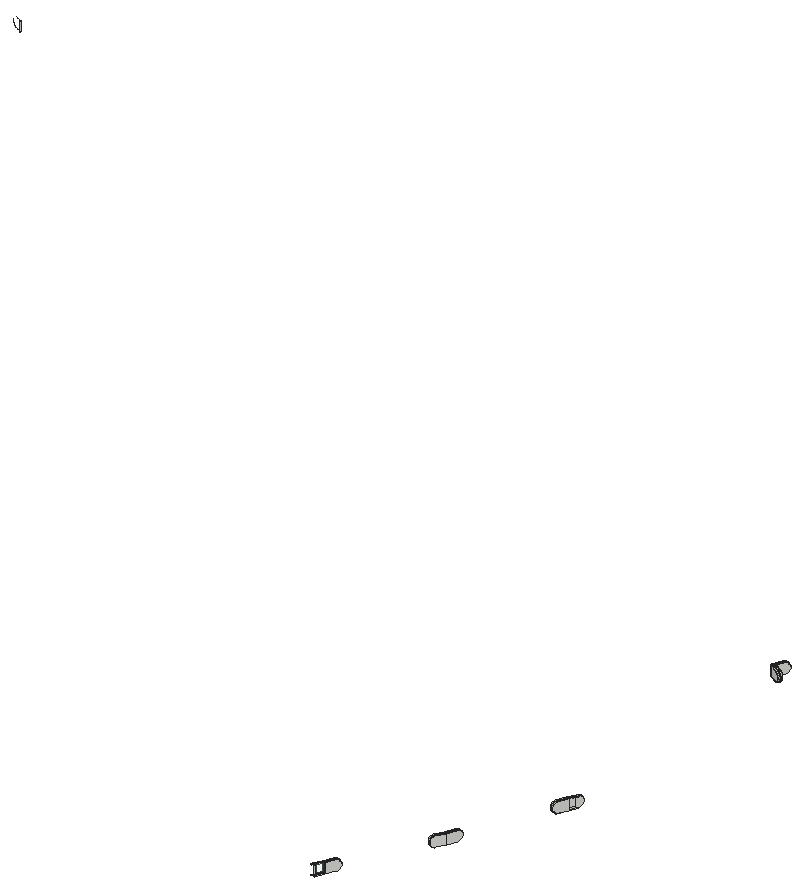
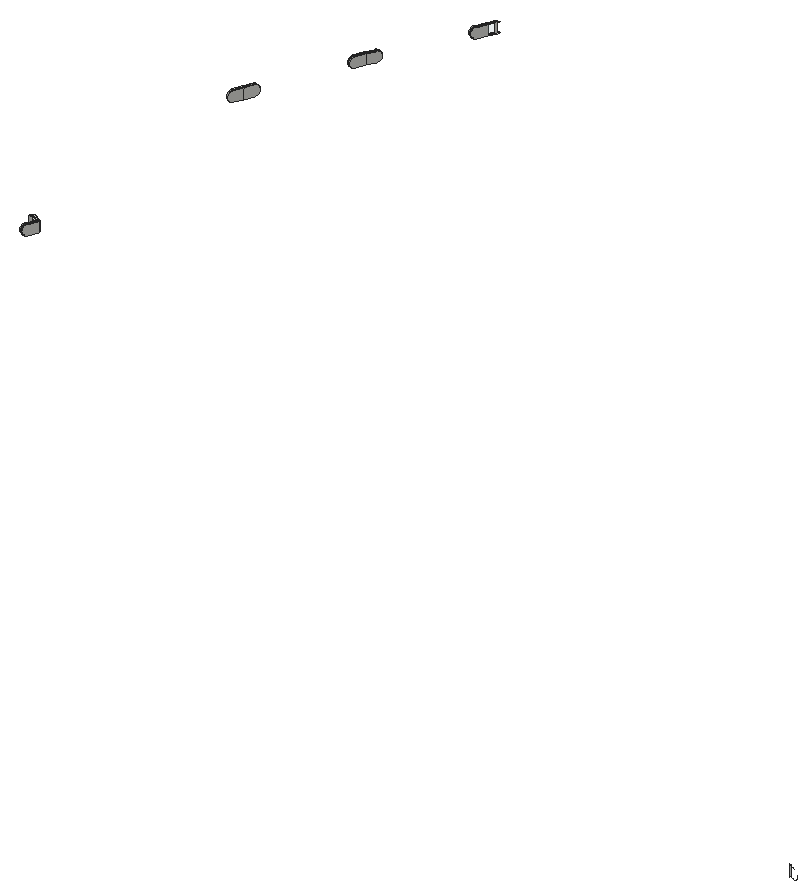
# SketchUp Ruby script. Lengths in inches.
U = 1.inch
M = Sketchup.active_model
def pt(a) = Geom::Point3d.new(a.map { |v| v * U })
def face(e, loops, mat)
  f = e.add_face(loops[0].map { |a| pt(a) })
  loops[1..].each { |l| e.add_face(l.map { |a| pt(a) }).erase! }
  f.material = f.back_material = mat if mat
  f
end
# faces: each face lists its corners as indices into pts; further lists are holes
def faces(e, pts, list, mat = nil) = list.each { |f| face(e, (f[0].is_a?(Array) ? f : [f]).map { |l| l.map { |i| pts[i] } }, mat) }
# xy, xz, yz: faces in a plane at the given z, y or x. An outline is a flat list of corners, or four numbers for a rectangle; further outlines are holes
def ring(l) = l.size == 4 ? [[l[0], l[1]], [l[2], l[1]], [l[2], l[3]], [l[0], l[3]]] : l.each_slice(2).to_a
def flat(e, list, mat, &to3) = list.each { |f| face(e, (f[0].is_a?(Array) ? f : [f]).map { |l| ring(l).map { |u, v| to3.(u, v) } }, mat) }
def xy(e, z, list, mat = nil) = flat(e, list, mat) { |x, y| [x, y, z] }
def xz(e, y, list, mat = nil) = flat(e, list, mat) { |x, z| [x, y, z] }
def yz(e, x, list, mat = nil) = flat(e, list, mat) { |y, z| [x, y, z] }
def lines(e, pts, list) = list.each { |a, b| e.add_line(pt(pts[a]), pt(pts[b])) }
# prism: a flat outline (further loops are holes) pulled along v
def prism(e, loops, v, mat = nil)
  f = face(e, loops, mat); d = Geom::Vector3d.new(v.map { |x| x * U })
  f.pushpull(f.normal.samedirection?(d) ? d.length : -d.length)
end
def box(e, o, s, mat = nil) = prism(e, [[o, [o[0] + s[0], o[1], o[2]], [o[0] + s[0], o[1] + s[1], o[2]], [o[0], o[1] + s[1], o[2]]]], [0, 0, s[2]], mat)
def at(x, y, z, deg = 0) = Geom::Transformation.translation(pt([x, y, z])) * Geom::Transformation.rotation(ORIGIN, Z_AXIS, deg.degrees)
def axes(o, x, y, z) = Geom::Transformation.new([*x, 0, *y, 0, *z, 0, *pt(o).to_a, 1])
def part(name) = M.definitions.add(name)
# library, detail: a bought-in or finely detailed component or shape, given as its bounding box
def library(name, o, s) = part(name).tap { |d| box(d.entities, o, s) }
def detail(e, o, s) = box(e.add_group.entities, o, s)
def put(e, d, t, mat = nil) = e.add_instance(d, t).tap { |i| i.material = mat if mat }
def group(e, t, mat = nil) = e.add_group.tap { |g| g.transformation = t; g.material = mat if mat }.entities
root = M.entities
M.materials.add("Glass_Safety_01").color = [204, 235, 244]
M.materials["Glass_Safety_01"].alpha = 0.1
M.materials.add("[Color_000]").color = [255, 255, 255]
xy(root,333,[[944.885,768.202,944.633,768.313,944.699,768.465,945.424,770.112,945.673,769.993],[944.452,768.392,944.2,768.503,944.993,770.305,945.245,770.194,944.519,768.544],[945.673,769.993,945.424,770.112,945.425,770.115,945.677,770.004,945.675,769.999],[945.677,770.004,945.425,770.115,946.271,771.889,946.52,771.77],[945.246,770.197,944.997,770.315,945.844,772.092,946.093,771.974],
  [954.439,788.385,954.19,788.504,954.265,788.661,955.037,790.281,955.286,790.162],[954.013,788.589,953.764,788.707,954.6,790.46,954.857,790.359,954.087,788.745],[955.297,790.187,955.04,790.287,955.76,792.12,956.016,792.019],[954.857,790.359,954.6,790.46,954.605,790.472,954.611,790.484,954.86,790.366],[954.86,790.366,954.611,790.484,955.32,792.292,955.577,792.192],
  [963.05,809.92,962.794,810.021,962.855,810.177,963.512,811.85,963.765,811.74],[962.61,810.093,962.354,810.194,963.074,812.026,963.33,811.925,962.671,810.249],[963.765,811.74,963.512,811.85,963.513,811.853,963.77,811.753,963.767,811.746],[963.77,811.753,963.513,811.853,964.298,813.655,964.551,813.545],[963.332,811.929,963.079,812.039,963.865,813.843,964.118,813.733],
  [963.328,866.978,961.618,867.953,961.755,868.193,963.309,867.306,963.464,867.217],[963.562,867.388,963.406,867.477,962.17,868.183,962.28,868.437,963.698,867.627],[962.146,868.129,961.894,868.239,961.929,868.32,962.04,868.574,962.68,870.044,962.932,869.934,962.28,868.437,962.04,868.574,961.989,868.603,961.852,868.364,961.929,868.32,962.17,868.183],[962.17,868.183,961.929,868.32,962.04,868.574,962.28,868.437],[961.713,868.317,961.46,868.428,962.246,870.232,962.499,870.122],
  [961.929,868.32,961.852,868.364,961.989,868.603,962.04,868.574]])
xy(root,333.078,[[944.791,768.673,944.611,768.752,945.245,770.194,945.335,770.154,945.424,770.112],[945.424,770.112,945.335,770.154,945.425,770.115,945.424,770.113],[945.425,770.115,945.335,770.154,945.246,770.197,945.924,771.618,946.101,771.534],[954.36,788.859,954.182,788.944,954.857,790.359,954.948,790.323,955.037,790.281],[955.04,790.287,954.948,790.323,954.86,790.366,955.433,791.825,955.616,791.753],
  [954.948,790.323,954.857,790.359,954.858,790.363,954.86,790.366],[962.9375,810.388,962.754,810.46,963.33,811.925,963.422,811.889,963.512,811.85],[963.512,811.85,963.422,811.889,963.513,811.853,963.513,811.852],[963.513,811.853,963.422,811.889,963.332,811.929,963.96,813.372,964.141,813.294],[963.122,867.412,961.755,868.193,961.803,868.278,961.894,868.239,961.929,868.32,963.22,867.583],
  [961.894,868.239,961.803,868.278,961.852,868.364,961.929,868.32],[961.803,868.278,961.713,868.317,962.342,869.761,962.522,869.683,961.929,868.32,961.852,868.364]],"Glass_Safety_01")
xy(root,335.047,[[944.791,768.673,945.424,770.112,945.335,770.154,945.245,770.194,944.611,768.752],[945.424,770.112,945.424,770.113,945.425,770.115,945.335,770.154],[945.425,770.115,946.101,771.534,945.924,771.618,945.246,770.197,945.335,770.154],[954.36,788.859,955.037,790.281,954.948,790.323,954.857,790.359,954.182,788.944],[955.04,790.287,955.616,791.753,955.433,791.825,954.86,790.366,954.948,790.323],
  [954.948,790.323,954.86,790.366,954.858,790.363,954.857,790.359],[962.9375,810.388,963.512,811.85,963.422,811.889,963.33,811.925,962.754,810.46],[963.512,811.85,963.513,811.852,963.513,811.853,963.422,811.889],[963.513,811.853,964.141,813.294,963.96,813.372,963.332,811.929,963.422,811.889],[963.122,867.412,963.22,867.583,961.929,868.32,961.894,868.239,961.803,868.278,961.755,868.193],
  [961.894,868.239,961.929,868.32,961.852,868.364,961.803,868.278],[961.803,868.278,961.852,868.364,961.929,868.32,962.522,869.683,962.342,869.761,961.713,868.317]],"Glass_Safety_01")
xy(root,335.126,[[944.885,768.202,945.673,769.993,945.424,770.112,944.699,768.465,944.633,768.313],[944.452,768.392,944.519,768.544,945.245,770.194,944.993,770.305,944.2,768.503],[945.673,769.993,945.675,769.999,945.677,770.004,945.425,770.115,945.424,770.112],[945.677,770.004,946.52,771.77,946.271,771.889,945.425,770.115],[945.246,770.197,946.093,771.974,945.844,772.092,944.997,770.315],
  [954.439,788.385,955.286,790.162,955.037,790.281,954.265,788.661,954.19,788.504],[954.013,788.589,954.087,788.745,954.857,790.359,954.6,790.46,953.764,788.707],[955.297,790.187,956.016,792.019,955.76,792.12,955.04,790.287],[954.857,790.359,954.86,790.366,954.611,790.484,954.605,790.472,954.6,790.46],[954.86,790.366,955.577,792.192,955.32,792.292,954.611,790.484],
  [963.05,809.92,963.765,811.74,963.512,811.85,962.855,810.177,962.794,810.021],[962.61,810.093,962.671,810.249,963.33,811.925,963.074,812.026,962.354,810.194],[963.765,811.74,963.767,811.746,963.77,811.753,963.513,811.853,963.512,811.85],[963.77,811.753,964.551,813.545,964.298,813.655,963.513,811.853],[963.332,811.929,964.118,813.733,963.865,813.843,963.079,812.039],
  [963.328,866.978,963.464,867.217,963.309,867.306,961.755,868.193,961.618,867.953],[963.562,867.388,963.698,867.627,962.28,868.437,962.17,868.183,963.406,867.477],[962.146,868.129,962.17,868.183,961.929,868.32,961.852,868.364,961.989,868.603,962.04,868.574,962.28,868.437,962.932,869.934,962.68,870.044,962.04,868.574,961.929,868.32,961.894,868.239],[962.17,868.183,962.28,868.437,962.04,868.574,961.929,868.32],[961.713,868.317,962.499,870.122,962.246,870.232,961.46,868.428],
  [961.929,868.32,962.04,868.574,961.989,868.603,961.852,868.364]])
p = [[944.452,768.392,333],[944.342,768.14,333.036],[944.089,768.251,333.036],[944.2,768.503,333],[945.245,770.194,335.126],[944.519,768.544,335.126],
  [944.519,768.544,333],[945.245,770.194,333],[945.245,770.194,333.078],[944.611,768.752,333.078],[944.611,768.752,335.047],[945.245,770.194,335.047],
  [945.424,770.112,333.078],[945.424,770.112,333],[945.673,769.993,333],[945.673,769.993,335.126],[945.424,770.112,335.126],[945.424,770.112,335.047],
  [945.425,770.115,333],[945.425,770.115,333.078],[945.425,770.115,335.047],[945.425,770.115,335.126],[945.677,770.004,335.126],[945.677,770.004,333],
  [945.675,769.999,335.126],[945.675,769.999,333],[946.52,771.77,333],[946.638,772.019,333.036],[946.748,772.25,333.142],[946.843,772.449,333.311],
  [946.916,772.601,333.531],[946.961,772.697,333.787],[946.977,772.73,334.0625],[946.961,772.697,334.338],[946.916,772.601,334.594],[946.843,772.449,334.814],
  [946.748,772.25,334.983],[946.638,772.019,335.089],[946.52,771.77,335.126],[946.271,771.889,335.126],[946.389,772.137,335.089],[946.5,772.369,334.983],
  [946.594,772.568,334.814],[946.667,772.72,334.594],[946.713,772.816,334.338],[946.728,772.849,334.0625],[946.713,772.816,333.787],[946.667,772.72,333.531],
  [946.594,772.568,333.311],[946.5,772.369,333.142],[946.389,772.137,333.036],[946.271,771.889,333],[944.993,770.305,333],[944.993,770.305,335.126],
  [945.246,770.197,333],[945.246,770.197,333.078],[945.246,770.197,335.047],[945.246,770.197,335.126],[944.997,770.315,335.126],[944.997,770.315,333],
  [946.093,771.974,333],[946.093,771.974,335.126],[945.924,771.618,335.047],[945.924,771.618,333.078],[945.844,772.092,335.126],[945.963,772.341,335.089],
  [946.073,772.572,334.983],[946.168,772.771,334.814],[946.24,772.923,334.594],[946.286,773.019,334.338],[946.302,773.052,334.0625],[946.286,773.019,333.787],
  [946.24,772.923,333.531],[946.168,772.771,333.311],[946.073,772.572,333.142],[945.963,772.341,333.036],[945.844,772.092,333],[946.211,772.222,333.036],
  [946.211,772.222,335.089],[946.322,772.454,334.983],[946.417,772.652,334.814],[946.489,772.805,334.594],[946.535,772.901,334.338],[946.55,772.933,334.0625],
  [946.535,772.901,333.787],[946.489,772.805,333.531],[946.417,772.652,333.311],[946.322,772.454,333.142],[955.286,790.162,335.126],[954.439,788.385,335.126],
  [954.321,788.137,335.089],[954.21,787.906,334.983],[954.116,787.707,334.814],[954.043,787.554,334.594],[953.997,787.459,334.338],[953.982,787.426,334.0625],
  [953.997,787.459,333.787],[954.043,787.554,333.531],[954.116,787.707,333.311],[954.21,787.906,333.142],[954.321,788.137,333.036],[954.439,788.385,333],
  [955.286,790.162,333],[954.19,788.504,335.126],[954.265,788.661,335.126],[954.265,788.661,333],[954.19,788.504,333],[954.072,788.256,333.036],
  [953.962,788.024,333.142],[953.867,787.826,333.311],[953.794,787.673,333.531],[953.748,787.577,333.787],[953.733,787.544,334.0625],[953.748,787.577,334.338],
  [953.794,787.673,334.594],[953.867,787.826,334.814],[953.962,788.024,334.983],[954.072,788.256,335.089],[954.013,788.589,333],[954.087,788.745,333],
  [954.857,790.359,333],[954.857,790.359,333.078],[954.857,790.359,335.047],[954.857,790.359,335.126],[954.087,788.745,335.126],[954.013,788.589,335.126],
  [953.894,788.34,335.089],[953.784,788.109,334.983],[953.689,787.91,334.814],[953.616,787.758,334.594],[953.571,787.662,334.338],[953.555,787.629,334.0625],
  [953.571,787.662,333.787],[953.616,787.758,333.531],[953.689,787.91,333.311],[953.784,788.109,333.142],[953.894,788.34,333.036],[953.764,788.707,335.126],
  [954.6,790.46,335.126],[954.6,790.46,333],[953.764,788.707,333],[953.645,788.459,333.036],[953.535,788.228,333.142],[953.44,788.029,333.311],
  [953.368,787.876,333.531],[953.322,787.78,333.787],[953.306,787.748,334.0625],[953.322,787.78,334.338],[953.368,787.876,334.594],[953.44,788.029,334.814],
  [953.535,788.228,334.983],[953.645,788.459,335.089],[955.037,790.281,333],[955.037,790.281,335.126],[955.037,790.281,335.047],[954.36,788.859,335.047],
  [954.36,788.859,333.078],[955.037,790.281,333.078],[955.04,790.287,333.078],[955.04,790.287,333],[955.297,790.187,333],[955.297,790.187,335.126],
  [955.04,790.287,335.126],[955.04,790.287,335.047],[956.016,792.019,335.126],[956.016,792.019,333],[956.117,792.275,333.036],[956.211,792.513,333.142],
  [956.291,792.718,333.311],[956.353,792.876,333.531],[956.392,792.974,333.787],[956.405,793.008,334.0625],[956.392,792.974,334.338],[956.353,792.876,334.594],
  [956.291,792.718,334.814],[956.211,792.513,334.983],[956.117,792.275,335.089],[955.76,792.12,335.126],[955.76,792.12,333],[955.616,791.753,333.078],
  [955.616,791.753,335.047],[954.86,790.366,333.078],[954.86,790.366,333],[954.611,790.484,333],[954.611,790.484,335.126],[954.86,790.366,335.126],
  [954.86,790.366,335.047],[955.577,792.192,333],[955.677,792.448,333.036],[955.771,792.686,333.142],[955.852,792.891,333.311],[955.913,793.048,333.531],
  [955.952,793.147,333.787],[955.965,793.181,334.0625],[955.952,793.147,334.338],[955.913,793.048,334.594],[955.852,792.891,334.814],[955.771,792.686,334.983],
  [955.677,792.448,335.089],[955.577,792.192,335.126],[954.605,790.472,333],[954.605,790.472,335.126],[955.32,792.292,335.126],[955.421,792.548,335.089],
  [955.515,792.787,334.983],[955.595,792.992,334.814],[955.657,793.149,334.594],[955.696,793.248,334.338],[955.709,793.282,334.0625],[955.696,793.248,333.787],
  [955.657,793.149,333.531],[955.595,792.992,333.311],[955.515,792.787,333.142],[955.421,792.548,333.036],[955.32,792.292,333],[955.86,792.376,333.036],
  [955.954,792.614,333.142],[956.035,792.819,333.311],[956.097,792.976,333.531],[956.135,793.075,333.787],[956.149,793.109,334.0625],[956.135,793.075,334.338],
  [956.097,792.976,334.594],[956.035,792.819,334.814],[955.954,792.614,334.983],[955.86,792.376,335.089],[963.05,809.92,333],[963.765,811.74,333],
  [963.765,811.74,335.126],[963.05,809.92,335.126],[962.949,809.664,335.089],[962.856,809.426,334.983],[962.775,809.221,334.814],[962.713,809.064,334.594],
  [962.675,808.965,334.338],[962.661,808.931,334.0625],[962.675,808.965,333.787],[962.713,809.064,333.531],[962.775,809.221,333.311],[962.856,809.426,333.142],
  [962.949,809.664,333.036],[962.855,810.177,335.126],[963.512,811.85,335.126],[963.512,811.85,335.047],[963.512,811.85,333.078],[963.512,811.85,333],
  [962.855,810.177,333],[962.794,810.021,333],[962.693,809.765,333.036],[962.599,809.527,333.142],[962.519,809.322,333.311],[962.457,809.164,333.531],
  [962.418,809.066,333.787],[962.405,809.032,334.0625],[962.418,809.066,334.338],[962.457,809.164,334.594],[962.519,809.322,334.814],[962.599,809.527,334.983],
  [962.693,809.765,335.089],[962.794,810.021,335.126],[962.61,810.093,333],[962.671,810.249,333],[962.671,810.249,335.126],[962.61,810.093,335.126],
  [962.51,809.837,335.089],[962.416,809.599,334.983],[962.335,809.394,334.814],[962.274,809.236,334.594],[962.235,809.138,334.338],[962.222,809.104,334.0625],
  [962.235,809.138,333.787],[962.274,809.236,333.531],[962.335,809.394,333.311],[962.416,809.599,333.142],[962.51,809.837,333.036],[962.354,810.194,335.126],
  [963.074,812.026,335.126],[963.074,812.026,333],[962.354,810.194,333],[962.253,809.938,333.036],[962.159,809.699,333.142],[962.079,809.494,333.311],
  [962.017,809.337,333.531],[961.978,809.238,333.787],[961.965,809.205,334.0625],[961.978,809.238,334.338],[962.017,809.337,334.594],[962.079,809.494,334.814],
  [962.159,809.699,334.983],[962.253,809.938,335.089],[963.33,811.925,335.126],[963.33,811.925,333],[963.33,811.925,333.078],[962.754,810.46,333.078],
  [962.754,810.46,335.047],[963.33,811.925,335.047],[963.767,811.746,335.126],[963.767,811.746,333],[963.77,811.753,333],[963.77,811.753,335.126],
  [963.513,811.853,333],[963.513,811.853,333.078],[963.513,811.853,335.047],[963.513,811.853,335.126],[963.332,811.929,333],[963.332,811.929,333.078],
  [963.332,811.929,335.047],[963.332,811.929,335.126],[963.079,812.039,335.126],[963.079,812.039,333],[964.118,813.733,333],[964.118,813.733,335.126],
  [963.96,813.372,335.047],[963.96,813.372,333.078],[964.298,813.655,335.126],[964.408,813.907,335.089],[964.51,814.142,334.983],[964.598,814.344,334.814],
  [964.666,814.499,334.594],[964.708,814.596,334.338],[964.723,814.629,334.0625],[964.708,814.596,333.787],[964.666,814.499,333.531],[964.598,814.344,333.311],
  [964.51,814.142,333.142],[964.408,813.907,333.036],[964.298,813.655,333],[963.865,813.843,335.126],[963.975,814.096,335.089],[964.077,814.331,334.983],
  [964.165,814.533,334.814],[964.232,814.6875,334.594],[964.275,814.785,334.338],[964.289,814.818,334.0625],[964.275,814.785,333.787],[964.232,814.6875,333.531],
  [964.165,814.533,333.311],[964.077,814.331,333.142],[963.975,814.096,333.036],[963.865,813.843,333],[964.227,813.986,333.036],[964.33,814.221,333.142],
  [963.328,866.978,335.126],[961.618,867.953,335.126],[961.618,867.953,333],[963.328,866.978,333],[963.567,866.841,333.036],[963.789,866.714,333.142],
  [963.981,866.605,333.311],[964.127,866.522,333.531],[964.22,866.469,333.787],[964.251,866.451,334.0625],[964.22,866.469,334.338],[964.127,866.522,334.594],
  [963.981,866.605,334.814],[963.789,866.714,334.983],[963.567,866.841,335.089],[963.464,867.217,333],[963.309,867.306,333],[963.309,867.306,335.126],
  [963.464,867.217,335.126],[963.703,867.081,335.089],[963.926,866.954,334.983],[964.117,866.845,334.814],[964.264,866.761,334.594],[964.356,866.708,334.338],
  [964.388,866.69,334.0625],[964.356,866.708,333.787],[964.264,866.761,333.531],[964.117,866.845,333.311],[963.926,866.954,333.142],[963.703,867.081,333.036],
  [963.562,867.388,335.126],[963.406,867.477,335.126],[963.406,867.477,333],[963.562,867.388,333],[963.801,867.252,333.036],[964.024,867.125,333.142],
  [964.215,867.016,333.311],[964.361,866.932,333.531],[964.454,866.879,333.787],[964.485,866.861,334.0625],[964.454,866.879,334.338],[964.361,866.932,334.594],
  [964.215,867.016,334.814],[964.024,867.125,334.983],[963.801,867.252,335.089],[961.989,868.603,335.126],[962.04,868.574,335.126],[962.28,868.437,335.126],
  [963.698,867.627,335.126],[963.9375,867.491,335.089],[964.16,867.364,334.983],[964.351,867.255,334.814],[964.498,867.171,334.594],[964.59,867.119,334.338],
  [964.622,867.101,334.0625],[964.59,867.119,333.787],[964.498,867.171,333.531],[964.351,867.255,333.311],[964.16,867.364,333.142],[963.9375,867.491,333.036],
  [963.698,867.627,333],[962.28,868.437,333],[962.04,868.574,333],[961.989,868.603,333],[961.755,868.193,335.126],[961.755,868.193,333],
  [961.755,868.193,333.078],[963.122,867.412,333.078],[963.122,867.412,335.047],[961.755,868.193,335.047],[962.17,868.183,333],[962.17,868.183,335.126],
  [961.929,868.32,335.126],[961.852,868.364,335.126],[961.852,868.364,335.047],[961.929,868.32,335.047],[963.22,867.583,335.047],[963.22,867.583,333.078],
  [961.929,868.32,333.078],[961.852,868.364,333.078],[961.852,868.364,333],[961.929,868.32,333],[961.894,868.239,333.078],[961.894,868.239,333],
  [962.146,868.129,333],[962.146,868.129,335.126],[961.894,868.239,335.126],[961.894,868.239,335.047],[962.932,869.934,333],[963.042,870.186,333.036],
  [963.145,870.421,333.142],[963.232,870.623,333.311],[963.3,870.778,333.531],[963.342,870.875,333.787],[963.357,870.908,334.0625],[963.342,870.875,334.338],
  [963.3,870.778,334.594],[963.232,870.623,334.814],[963.145,870.421,334.983],[963.042,870.186,335.089],[962.932,869.934,335.126],[962.68,870.044,335.126],
  [962.68,870.044,333],[962.522,869.683,333.078],[962.522,869.683,335.047],[961.713,868.317,333],[961.713,868.317,333.078],[961.713,868.317,335.047],
  [961.713,868.317,335.126],[961.46,868.428,335.126],[961.46,868.428,333],[962.499,870.122,333],[962.499,870.122,335.126],[962.342,869.761,335.047],
  [962.342,869.761,333.078],[962.246,870.232,335.126],[962.356,870.485,335.089],[962.459,870.72,334.983],[962.547,870.921,334.814],[962.614,871.076,334.594],
  [962.656,871.174,334.338],[962.671,871.207,334.0625],[962.656,871.174,333.787],[962.614,871.076,333.531],[962.547,870.921,333.311],[962.459,870.72,333.142],
  [962.356,870.485,333.036],[962.246,870.232,333],[962.789,870.296,333.036],[962.892,870.531,333.142],[962.98,870.733,333.311],[963.047,870.888,333.531],
  [963.09,870.985,333.787],[963.104,871.018,334.0625],[963.09,870.985,334.338],[963.047,870.888,334.594],[962.98,870.733,334.814],[962.892,870.531,334.983],
  [962.789,870.296,335.089],[962.609,870.374,333.036],[962.609,870.374,335.089],[962.711,870.61,334.983],[962.799,870.811,334.814],[962.867,870.966,334.594],
  [962.909,871.064,334.338],[962.924,871.097,334.0625],[962.909,871.064,333.787],[962.867,870.966,333.531],[962.799,870.811,333.311],[962.711,870.61,333.142],
  [729.122,960.111,335.126],[729.122,960.111,333],[729.137,960.039,333],[729.137,960.039,335.126],[944.791,768.673,333.078],[944.791,768.673,335.047],
  [945.335,770.154,335.047],[945.335,770.154,333.078],[945.424,770.113,333.078],[945.424,770.113,335.047],[946.101,771.534,335.047],[946.101,771.534,333.078],
  [954.182,788.944,335.047],[954.182,788.944,333.078],[954.948,790.323,333.078],[954.948,790.323,335.047],[954.858,790.363,335.047],[954.858,790.363,333.078],
  [955.433,791.825,333.078],[955.433,791.825,335.047],[962.9375,810.388,333.078],[962.9375,810.388,335.047],[963.422,811.889,335.047],[963.422,811.889,333.078],
  [963.513,811.852,333.078],[963.513,811.852,335.047],[964.141,813.294,335.047],[964.141,813.294,333.078],[964.418,814.423,333.311],[961.803,868.278,335.047],
  [961.803,868.278,333.078],[964.227,813.986,335.089],[964.33,814.221,334.983],[944.342,768.14,335.089],[944.452,768.392,335.126],[944.2,768.503,335.126],
  [944.089,768.251,335.089],[726.893,961.128,334.338],[726.86,961.144,334.0625],[726.893,961.128,333.787],[726.988,961.082,333.531],[727.14,961.008,333.311],
  [727.338,960.912,333.142],[727.569,960.8,333.036],[727.816,960.68,333],[729.587,959.82,335.126],[727.816,960.68,335.126]]
faces(root,p,[[0,1,2,3],[4,5,6,7,8,9,10,11],[12,13,14,15,16,17],[18,19,20,21,22,23],[24,15,14,25,23,22],[24,15,14,25,23,26,27,28,29,30,31,32,33,34,35,36,37,38,22],[18,13,12,17,16,21,20,19],[16,21,39,40,41,42,43,44,45,46,47,48,49,50,51,18,13,12,17],
  [8,7,52,53,4,11],[54,55,56,57,58,59],[54,60,61,57,56,62,63,55],[58,64,65,66,67,68,69,70,71,72,73,74,75,76,59],[51,50,27,26],[77,60,76,75],[50,49,28,27],[87,77,75,74],
  [88,89,90,91,92,93,94,95,96,97,98,99,100,101,102],[103,104,105,106,107,108,109,110,111,112,113,114,115,116,117],[118,119,120,121,122,123,124,125,126,127,128,129,130,131,132,133,134,135,136],[137,138,139,140,141,142,143,144,145,146,147,148,149,150,151],[108,107,100,99],[136,135,142,141],[107,106,101,100],[118,136,141,140],
  [152,105,104,153,154,155,156,157],[152,157,154,153,88,102],[158,159,160,161,162,163],[164,161,160,165,166,167,168,169,170,171,172,173,174,175,176],[162,177,178,159,158,179,180,163],[120,121,122,123,138,139],[181,182,183,184,185,186],[185,123,122,121,120,182,181,186],
  [185,123,122,121,120,182,187,188,189,190,191,192,193,194,195,196,197,198,199],[200,139,138,201,184,183],[138,201,184,202,203,204,205,206,207,208,209,210,211,212,213,214,183,200,139],[178,215,166,165],[188,187,214,213],[215,216,167,166],[189,188,213,212],[226,227,228,229,230,231,232,233,234,235,236,237,238,239,240],
  [241,242,243,244,245,246,247,248,249,250,251,252,253,254,255,256,257,258,259],[260,261,262,263,264,265,266,267,268,269,270,271,272,273,274],[275,276,277,278,279,280,281,282,283,284,285,286,287,288,289],[249,248,240,239],[274,273,280,279],[248,247,226,240],[260,274,279,278],[290,262,261,291,292,293,294,295],
  [244,245,227,228,242,243],[296,228,227,297,298,299],[300,301,302,303,299,298],[292,291,277,276,290,295],[304,305,306,307,308,309],[304,310,311,307,306,312,313,305],[300,245,244,243,242,303,302,301],[242,303,314,315,316,317,318,319,320,321,322,323,324,325,326,300,245,244,243],
  [308,327,328,329,330,331,332,333,334,335,336,337,338,339,309],[340,310,339,338],[341,340,338,337],[342,343,344,345,346,347,348,349,350,351,352,353,354,355,356],[357,358,359,360,361,362,363,364,365,366,367,368,369,370,371],[371,370,347,346],[357,371,346,345],[372,373,374,375,376,377,378,379,380,381,382,383,384,385,386],
  [387,388,389,390,391,392,393,394,395,396,397,398,399,400,401,402,403,404,405],[377,376,401,400],[406,359,358,407,408,409,410,411],[376,375,402,401],[412,374,373,413,414,415,416,417,418,419,420,421,422,423],[408,407,344,343,406,411],[424,425,426,427,428,429],[413,427,426,412,403,430,431,432,433,434,435,436,437,438,439,440,441,442,389],
  [388,443,444,404,423,425,424,420,445,446,417,429,428,414],[447,448,449,450,451,452],[447,453,454,450,449,455,456,448],[451,457,458,459,460,461,462,463,464,465,466,467,468,469,452],[422,421,416,415,387,405],[444,470,431,430],[481,453,469,468],[470,471,432,431],
  [491,481,468,467],[49,48,29,28],[86,87,74,73],[109,108,99,98],[135,134,143,142],[216,217,168,167],[190,189,212,211],[250,249,239,238],
  [273,272,281,280],[520,341,337,336],[370,369,348,347],[378,377,400,399],[471,472,433,432],[490,491,467,466],[48,47,30,29],[85,86,73,72],
  [110,109,98,97],[134,133,144,143],[217,218,169,168],[191,190,211,210],[251,250,238,237],[272,271,282,281],[369,368,349,348],[472,473,434,433],
  [489,490,466,465],[47,46,31,30],[84,85,72,71],[111,110,97,96],[133,132,145,144],[218,219,170,169],[192,191,210,209],[252,251,237,236],
  [271,270,283,282],[368,367,350,349],[473,474,435,434],[488,489,465,464],[46,45,32,31],[83,84,71,70],[112,111,96,95],[132,131,146,145],
  [219,220,171,170],[193,192,209,208],[253,252,236,235],[270,269,284,283],[474,475,436,435],[487,488,464,463],[45,44,33,32],[82,83,70,69],
  [113,112,95,94],[131,130,147,146],[220,221,172,171],[194,193,208,207],[254,253,235,234],[269,268,285,284],[475,476,437,436],[486,487,463,462],
  [44,43,34,33],[81,82,69,68],[114,113,94,93],[130,129,148,147],[221,222,173,172],[195,194,207,206],[255,254,234,233],[268,267,286,285],
  [365,364,353,352],[476,477,438,437],[485,486,462,461],[43,42,35,34],[80,81,68,67],[115,114,93,92],[129,128,149,148],[222,223,174,173],
  [196,195,206,205],[256,255,233,232],[267,266,287,286],[364,363,354,353],[477,478,439,438],[484,485,461,460],[42,41,36,35],[79,80,67,66],
  [116,115,92,91],[128,127,150,149],[223,224,175,174],[197,196,205,204],[257,256,232,231],[266,265,288,287],[363,362,355,354],[385,384,393,392],
  [478,479,440,439],[483,484,460,459],[41,40,37,36],[78,79,66,65],[117,116,91,90],[127,126,151,150],[224,225,176,175],[198,197,204,203],
  [258,257,231,230],[265,264,289,288],[523,524,329,328],[362,361,356,355],[386,385,392,391],[479,480,441,440],[482,483,459,458],[525,526,527,528],
  [40,39,38,37],[61,78,65,64],[103,117,90,89],[126,125,137,151],[225,177,164,176],[199,198,203,202],[259,258,230,229],[264,263,275,289],
  [311,523,328,327],[361,360,342,356],[372,386,391,390],[480,443,442,441],[454,482,458,457]])
faces(root,p,[[39,51,50,49,48,47,46,45,44,43,42,41,40],[60,61,78,79,80,81,82,83,84,85,86,87,77],[177,178,215,216,217,218,219,220,221,222,223,224,225],[187,199,198,197,196,195,194,193,192,191,190,189,188],[443,444,470,471,472,473,474,475,476,477,478,479,480],[453,454,482,483,484,485,486,487,488,489,490,491,481],[496,497,10,9],[496,12,17,497],
  [9,8,11,10],[498,499,12,17],[19,499,498,20],[500,19,20,501,17,12],[502,20,19,503],[11,498,499,8],[499,498,56,55],[55,63,62,56],
  [62,502,503,63],[156,155,504,505],[504,122,121,505],[157,156,155,154],[506,507,122,121],[186,507,506,181],[157,506,507,154],[507,506,158,163],
  [179,158,163,180],[508,186,181,509,121,122],[510,181,186,511],[179,510,511,180],[512,513,294,293],[512,244,243,513],[293,292,295,294],[295,514,515,292],
  [515,514,306,305],[305,313,312,306],[514,515,244,243],[301,515,514,302],[516,301,302,517,243,244],[518,302,301,519],[312,518,519,313],[409,408,411,410],
  [419,418,410,409],[421,420,419,418,417,416],[411,521,522,408],[521,522,424,429],[420,424,429,417,446,445],[522,521,449,448],[448,456,455,449],[421,522,521,416],
  [455,446,445,456]],"Glass_Safety_01")
faces(root,p,[[492,493,494,495]],"[Color_000]")
lines(root,p,[[529,530],[530,531],[531,532],[532,533],[533,534],[534,535],[535,536],[536,494],[537,495],[495,538]])
